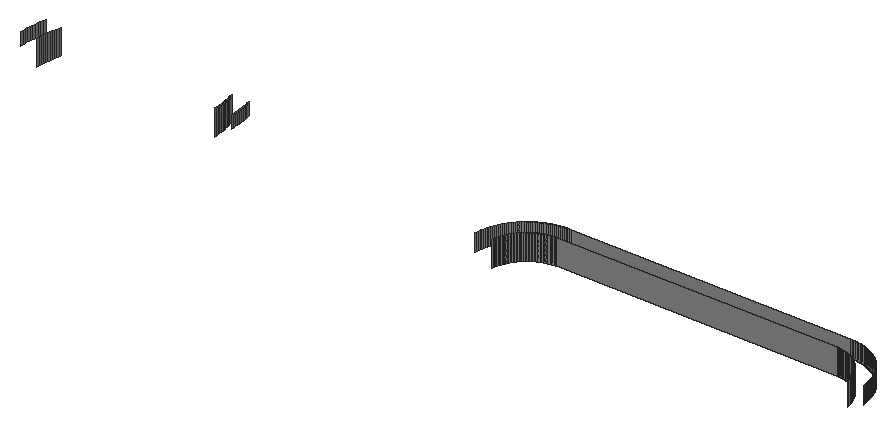
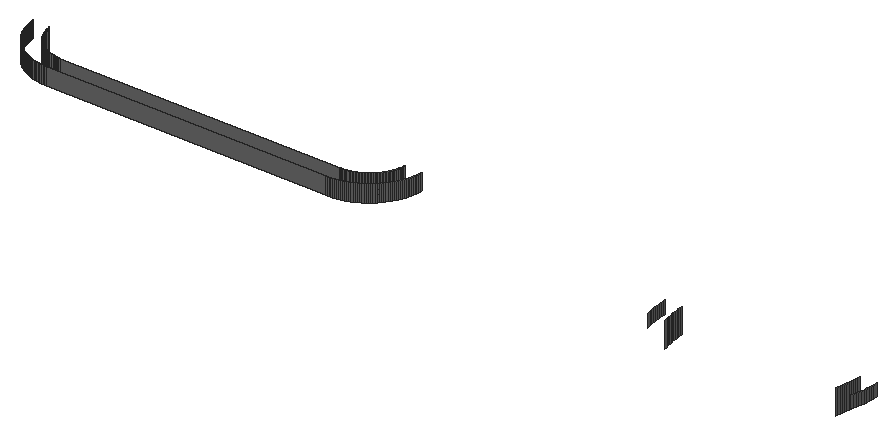
# SketchUp Ruby script. Lengths in inches.
U = 1.inch
M = Sketchup.active_model
def pt(a) = Geom::Point3d.new(a.map { |v| v * U })
def face(e, loops, mat)
  f = e.add_face(loops[0].map { |a| pt(a) })
  loops[1..].each { |l| e.add_face(l.map { |a| pt(a) }).erase! }
  f.material = f.back_material = mat if mat
  f
end
# faces: each face lists its corners as indices into pts; further lists are holes
def faces(e, pts, list, mat = nil) = list.each { |f| face(e, (f[0].is_a?(Array) ? f : [f]).map { |l| l.map { |i| pts[i] } }, mat) }
# xy, xz, yz: faces in a plane at the given z, y or x. An outline is a flat list of corners, or four numbers for a rectangle; further outlines are holes
def ring(l) = l.size == 4 ? [[l[0], l[1]], [l[2], l[1]], [l[2], l[3]], [l[0], l[3]]] : l.each_slice(2).to_a
def flat(e, list, mat, &to3) = list.each { |f| face(e, (f[0].is_a?(Array) ? f : [f]).map { |l| ring(l).map { |u, v| to3.(u, v) } }, mat) }
def xy(e, z, list, mat = nil) = flat(e, list, mat) { |x, y| [x, y, z] }
def xz(e, y, list, mat = nil) = flat(e, list, mat) { |x, z| [x, y, z] }
def yz(e, x, list, mat = nil) = flat(e, list, mat) { |y, z| [x, y, z] }
def lines(e, pts, list) = list.each { |a, b| e.add_line(pt(pts[a]), pt(pts[b])) }
# prism: a flat outline (further loops are holes) pulled along v
def prism(e, loops, v, mat = nil)
  f = face(e, loops, mat); d = Geom::Vector3d.new(v.map { |x| x * U })
  f.pushpull(f.normal.samedirection?(d) ? d.length : -d.length)
end
def box(e, o, s, mat = nil) = prism(e, [[o, [o[0] + s[0], o[1], o[2]], [o[0] + s[0], o[1] + s[1], o[2]], [o[0], o[1] + s[1], o[2]]]], [0, 0, s[2]], mat)
def at(x, y, z, deg = 0) = Geom::Transformation.translation(pt([x, y, z])) * Geom::Transformation.rotation(ORIGIN, Z_AXIS, deg.degrees)
def axes(o, x, y, z) = Geom::Transformation.new([*x, 0, *y, 0, *z, 0, *pt(o).to_a, 1])
def part(name) = M.definitions.add(name)
# library, detail: a bought-in or finely detailed component or shape, given as its bounding box
def library(name, o, s) = part(name).tap { |d| box(d.entities, o, s) }
def detail(e, o, s) = box(e.add_group.entities, o, s)
def put(e, d, t, mat = nil) = e.add_instance(d, t).tap { |i| i.material = mat if mat }
def group(e, t, mat = nil) = e.add_group.tap { |g| g.transformation = t; g.material = mat if mat }.entities
root = M.entities
M.materials.add("[Slate Light Tile]").color = [119, 119, 119]
M.materials.add("[Stone Coursed Rough]").color = [137, 137, 137]
xz(root,120,[[290.72,-2,291,4],[291,-2,357,4],[357,-2,357.28,4]],"[Stone Coursed Rough]")
xz(root,124,[[291,0,357,4]],"[Stone Coursed Rough]")
p = [[168.01,120.55,-3],[168.01,120.55,3],[168,120,3],[168,120,-3],[210,120,-3],[210,120,3],
  [209.99,120.55,3],[209.99,120.55,-3],[168.03,121.1,-3],[168.03,121.1,3],[209.97,121.1,3],[209.97,121.1,-3],
  [168.06,121.65,-3],[168.06,121.65,3],[209.94,121.65,3],[209.94,121.65,-3],[168.12,122.2,-3],[168.12,122.2,3],
  [209.88,122.2,3],[209.88,122.2,-3],[168.18,122.74,-3],[168.18,122.74,3],[209.82,122.74,3],[209.82,122.74,-3],
  [168.26,123.29,-3],[168.26,123.29,3],[209.74,123.29,3],[209.74,123.29,-3],[168.35,123.83,-3],[168.35,123.83,3],
  [209.65,123.83,3],[209.65,123.83,-3],[168.46,124.37,-3],[168.46,124.37,3],[209.54,124.37,3],[209.54,124.37,-3],
  [168.58,124.9,-3],[168.58,124.9,3],[209.42,124.9,3],[209.42,124.9,-3],[168.72,125.44,-3],[168.72,125.44,3],
  [209.28,125.44,3],[209.28,125.44,-3],[168.86,125.96,-3],[168.86,125.96,3],[209.14,125.96,3],[209.14,125.96,-3],
  [282.04,111.85,-2],[282.07,112.13,-2],[282.07,112.13,4],[282.04,111.85,4],[282.11,112.41,-2],[282.11,112.41,4],
  [365.89,112.41,-2],[365.93,112.13,-2],[365.93,112.13,4],[365.89,112.41,4],[282.16,112.6875,-2],[282.16,112.6875,4],
  [365.84,112.6875,-2],[365.84,112.6875,4],[282.22,112.96,-2],[282.22,112.96,4],[365.78,112.96,-2],[365.78,112.96,4],
  [282.28,113.24,-2],[282.28,113.24,4],[365.72,113.24,-2],[365.72,113.24,4],[282.36,113.51,-2],[282.36,113.51,4],
  [365.64,113.51,-2],[365.64,113.51,4],[282.44,113.78,-2],[282.44,113.78,4],[365.56,113.78,-2],[365.56,113.78,4],
  [282.53,114.05,-2],[282.53,114.05,4],[365.47,114.05,-2],[365.47,114.05,4],[282.63,114.3125,-2],[282.63,114.3125,4],
  [365.37,114.3125,-2],[365.37,114.3125,4],[282.74,114.57,-2],[282.74,114.57,4],[365.26,114.57,-2],[365.26,114.57,4],
  [282.86,114.83,-2],[282.86,114.83,4],[365.14,114.83,-2],[365.14,114.83,4],[282.98,115.09,-2],[282.98,115.09,4],
  [365.02,115.09,-2],[365.02,115.09,4],[283.11,115.34,-2],[283.11,115.34,4],[364.89,115.34,-2],[364.89,115.34,4],
  [283.25,115.58,-2],[283.25,115.58,4],[364.75,115.58,-2],[364.75,115.58,4],[283.4,115.82,-2],[283.4,115.82,4],
  [364.6,115.82,-2],[364.6,115.82,4],[283.56,116.06,-2],[283.56,116.06,4],[364.44,116.06,-2],[364.44,116.06,4],
  [283.72,116.29,-2],[283.72,116.29,4],[364.28,116.29,-2],[364.28,116.29,4],[283.89,116.52,-2],[283.89,116.52,4],
  [364.11,116.52,-2],[364.11,116.52,4],[284.07,116.74,-2],[284.07,116.74,4],[363.93,116.74,-2],[363.93,116.74,4],
  [284.25,116.95,-2],[284.25,116.95,4],[363.75,116.95,-2],[363.75,116.95,4],[284.4375,117.16,-2],[284.4375,117.16,4],
  [363.5625,117.16,-2],[363.5625,117.16,4],[284.64,117.36,-2],[284.64,117.36,4],[363.36,117.36,-2],[363.36,117.36,4],
  [284.84,117.5625,-2],[284.84,117.5625,4],[363.16,117.5625,-2],[363.16,117.5625,4],[285.05,117.75,-2],[285.05,117.75,4],
  [362.95,117.75,-2],[362.95,117.75,4],[285.26,117.93,-2],[285.26,117.93,4],[362.74,117.93,-2],[362.74,117.93,4],
  [285.48,118.11,-2],[285.48,118.11,4],[362.52,118.11,-2],[362.52,118.11,4],[285.71,118.28,-2],[285.71,118.28,4],
  [362.29,118.28,-2],[362.29,118.28,4],[285.94,118.44,-2],[285.94,118.44,4],[362.06,118.44,-2],[362.06,118.44,4],
  [286.18,118.6,-2],[286.18,118.6,4],[361.82,118.6,-2],[361.82,118.6,4],[286.42,118.75,-2],[286.42,118.75,4],
  [361.58,118.75,-2],[361.58,118.75,4],[286.66,118.89,-2],[286.66,118.89,4],[361.34,118.89,-2],[361.34,118.89,4],
  [286.91,119.02,-2],[286.91,119.02,4],[361.09,119.02,-2],[361.09,119.02,4],[287.17,119.14,-2],[287.17,119.14,4],
  [360.83,119.14,-2],[360.83,119.14,4],[287.43,119.26,-2],[287.43,119.26,4],[360.57,119.26,-2],[360.57,119.26,4],
  [287.6875,119.37,-2],[287.6875,119.37,4],[360.3125,119.37,-2],[360.3125,119.37,4],[287.95,119.47,-2],[287.95,119.47,4],
  [360.05,119.47,-2],[360.05,119.47,4],[288.22,119.56,-2],[288.22,119.56,4],[359.78,119.56,-2],[359.78,119.56,4],
  [288.49,119.64,-2],[288.49,119.64,4],[288.76,119.72,-2],[288.76,119.72,4],[359.24,119.72,-2],[359.51,119.64,-2],
  [359.51,119.64,4],[359.24,119.72,4],[289.04,119.78,-2],[289.04,119.78,4],[358.96,119.78,-2],[358.96,119.78,4],
  [289.3125,119.84,-2],[289.3125,119.84,4],[289.59,119.89,-2],[289.59,119.89,4],[358.41,119.89,-2],[358.6875,119.84,-2],
  [358.6875,119.84,4],[358.41,119.89,4],[289.87,119.93,-2],[289.87,119.93,4],[290.15,119.96,-2],[290.15,119.96,4],
  [357.85,119.96,-2],[358.13,119.93,-2],[358.13,119.93,4],[357.85,119.96,4],[290.43,119.98,-2],[290.43,119.98,4],
  [290.72,120,-2],[290.72,120,4],[357.28,120,-2],[357.57,119.98,-2],[357.57,119.98,4],[357.28,120,4],
  [278.06,112.22,0],[278.03,111.82,0],[278.03,111.82,4],[278.06,112.22,4],[369.97,111.82,0],[369.94,112.22,0],
  [369.94,112.22,4],[369.97,111.82,4],[278.1,112.63,0],[278.1,112.63,4],[369.9,112.63,0],[369.9,112.63,4],
  [278.16,113.03,0],[278.16,113.03,4],[369.84,113.03,0],[369.84,113.03,4],[278.23,113.4375,0],[278.23,113.4375,4],
  [369.77,113.4375,0],[369.77,113.4375,4],[278.3125,113.84,0],[278.3125,113.84,4],[369.6875,113.84,0],[369.6875,113.84,4],
  [278.41,114.23,0],[278.41,114.23,4],[369.59,114.23,0],[369.59,114.23,4],[278.52,114.625,0],[278.52,114.625,4],
  [369.48,114.625,0],[369.48,114.625,4],[278.64,115.02,0],[278.64,115.02,4],[369.36,115.02,0],[369.36,115.02,4],
  [278.77,115.4,0],[278.77,115.4,4],[369.23,115.4,0],[369.23,115.4,4],[278.91,115.79,0],[278.91,115.79,4],
  [369.09,115.79,0],[369.09,115.79,4],[279.07,116.16,0],[279.07,116.16,4],[368.93,116.16,0],[368.93,116.16,4],
  [279.24,116.54,0],[279.24,116.54,4],[368.76,116.54,0],[368.76,116.54,4],[279.42,116.9,0],[279.42,116.9,4],
  [368.58,116.9,0],[368.58,116.9,4],[279.61,117.26,0],[279.61,117.26,4],[368.39,117.26,0],[368.39,117.26,4],
  [279.81,117.62,0],[279.81,117.62,4],[368.19,117.62,0],[368.19,117.62,4],[280.02,117.97,0],[280.02,117.97,4],
  [367.98,117.97,0],[367.98,117.97,4],[280.25,118.31,0],[280.25,118.31,4],[367.75,118.31,0],[367.75,118.31,4],
  [280.48,118.64,0],[280.48,118.64,4],[367.52,118.64,0],[367.52,118.64,4],[280.73,118.97,0],[280.73,118.97,4],
  [367.27,118.97,0],[367.27,118.97,4],[280.98,119.29,0],[280.98,119.29,4],[367.02,119.29,0],[367.02,119.29,4],
  [281.25,119.6,0],[281.25,119.6,4],[366.75,119.6,0],[366.75,119.6,4],[281.52,119.9,0],[281.52,119.9,4],
  [366.48,119.9,0],[366.48,119.9,4],[281.81,120.19,0],[281.81,120.19,4],[366.19,120.19,0],[366.19,120.19,4],
  [164.01,120.65,0],[164,120,0],[164,120,3],[164.01,120.65,3],[214,120,0],[213.99,120.65,0],
  [213.99,120.65,3],[214,120,3],[282.1,120.48,0],[282.1,120.48,4],[365.9,120.48,0],[365.9,120.48,4],
  [282.4,120.75,0],[282.4,120.75,4],[365.6,120.75,0],[365.6,120.75,4],[164.03,121.31,0],[164.03,121.31,3],
  [213.97,121.31,0],[213.97,121.31,3],[282.71,121.02,0],[282.71,121.02,4],[365.29,121.02,0],[365.29,121.02,4],
  [283.03,121.27,0],[283.03,121.27,4],[364.97,121.27,0],[364.97,121.27,4],[164.08,121.96,0],[164.08,121.96,3],
  [213.92,121.96,0],[213.92,121.96,3],[283.36,121.52,0],[283.36,121.52,4],[364.64,121.52,0],[364.64,121.52,4],
  [283.69,121.75,0],[283.69,121.75,4],[364.31,121.75,0],[364.31,121.75,4],[284.03,121.98,0],[284.03,121.98,4],
  [363.97,121.98,0],[363.97,121.98,4],[164.14,122.61,0],[164.14,122.61,3],[213.86,122.61,0],[213.86,122.61,3],
  [284.38,122.19,0],[284.38,122.19,4],[363.62,122.19,0],[363.62,122.19,4],[284.74,122.39,0],[284.74,122.39,4],
  [363.26,122.39,0],[363.26,122.39,4],[285.1,122.58,0],[285.1,122.58,4],[362.9,122.58,0],[362.9,122.58,4],
  [164.21,123.26,0],[164.21,123.26,3],[213.79,123.26,0],[213.79,123.26,3],[285.46,122.76,0],[285.46,122.76,4],
  [362.54,122.76,0],[362.54,122.76,4],[285.84,122.93,0],[285.84,122.93,4],[362.16,122.93,0],[362.16,122.93,4],
  [286.21,123.09,0],[286.21,123.09,4],[361.79,123.09,0],[361.79,123.09,4],[286.6,123.23,0],[286.6,123.23,4],
  [361.4,123.23,0],[361.4,123.23,4],[286.98,123.36,0],[286.98,123.36,4],[361.02,123.36,0],[361.02,123.36,4],
  [164.31,123.91,0],[164.31,123.91,3],[213.69,123.91,0],[213.69,123.91,3],[287.375,123.48,0],[287.375,123.48,4],
  [360.625,123.48,0],[360.625,123.48,4],[287.77,123.59,0],[287.77,123.59,4],[360.23,123.59,0],[360.23,123.59,4],
  [288.16,123.6875,0],[288.16,123.6875,4],[359.84,123.6875,0],[359.84,123.6875,4],[288.5625,123.77,0],[288.5625,123.77,4],
  [359.4375,123.77,0],[359.4375,123.77,4],[288.97,123.84,0],[288.97,123.84,4],[289.37,123.9,0],[289.37,123.9,4],
  [359.03,123.84,0],[358.63,123.9,0],[358.63,123.9,4],[359.03,123.84,4],[164.42,124.56,0],[164.42,124.56,3],
  [213.58,124.56,0],[213.58,124.56,3],[289.78,123.94,0],[289.78,123.94,4],[290.18,123.97,0],[290.18,123.97,4],
  [358.22,123.94,0],[357.82,123.97,0],[357.82,123.97,4],[358.22,123.94,4],[290.59,123.99,0],[290.59,123.99,4],
  [291,124,0],[291,124,4],[357.41,123.99,0],[357,124,0],[357,124,4],[357.41,123.99,4],
  [164.55,125.2,0],[164.55,125.2,3],[213.45,125.2,0],[213.45,125.2,3],[164.69,125.84,0],[164.69,125.84,3],
  [213.31,125.84,0],[213.31,125.84,3],[164.85,126.47,0],[164.85,126.47,3]]
faces(root,p,[[0,1,2,3],[4,5,6,7],[8,9,1,0],[7,6,10,11],[12,13,9,8],[11,10,14,15],[16,17,13,12],[15,14,18,19],
  [20,21,17,16],[19,18,22,23],[24,25,21,20],[23,22,26,27],[28,29,25,24],[27,26,30,31],[32,33,29,28],[31,30,34,35],
  [36,37,33,32],[35,34,38,39],[40,41,37,36],[39,38,42,43],[44,45,41,40],[43,42,46,47],[330,331,332,333],[334,335,336,337],
  [346,330,333,347],[335,348,349,336],[358,346,347,359],[348,360,361,349],[374,358,359,375],[360,376,377,361],[390,374,375,391],[376,392,393,377],
  [414,390,391,415],[392,416,417,393],[442,414,415,443],[416,444,445,417],[462,442,443,463],[444,464,465,445],[466,462,463,467],[464,468,469,465],
  [470,466,467,471]],"[Slate Light Tile]")
faces(root,p,[[48,49,50,51],[49,52,53,50],[54,55,56,57],[52,58,59,53],[60,54,57,61],[58,62,63,59],[64,60,61,65],[62,66,67,63],
  [68,64,65,69],[66,70,71,67],[72,68,69,73],[70,74,75,71],[76,72,73,77],[74,78,79,75],[80,76,77,81],[78,82,83,79],
  [84,80,81,85],[82,86,87,83],[88,84,85,89],[86,90,91,87],[92,88,89,93],[90,94,95,91],[96,92,93,97],[94,98,99,95],
  [100,96,97,101],[98,102,103,99],[104,100,101,105],[102,106,107,103],[108,104,105,109],[106,110,111,107],[112,108,109,113],[110,114,115,111],
  [116,112,113,117],[114,118,119,115],[120,116,117,121],[118,122,123,119],[124,120,121,125],[122,126,127,123],[128,124,125,129],[126,130,131,127],
  [132,128,129,133],[130,134,135,131],[136,132,133,137],[134,138,139,135],[140,136,137,141],[138,142,143,139],[144,140,141,145],[142,146,147,143],
  [148,144,145,149],[146,150,151,147],[152,148,149,153],[150,154,155,151],[156,152,153,157],[154,158,159,155],[160,156,157,161],[158,162,163,159],
  [164,160,161,165],[162,166,167,163],[168,164,165,169],[166,170,171,167],[172,168,169,173],[170,174,175,171],[176,172,173,177],[174,178,179,175],
  [180,176,177,181],[178,182,183,179],[184,180,181,185],[182,186,187,183],[188,184,185,189],[186,190,191,187],[192,188,189,193],[190,194,195,191],
  [196,192,193,197],[194,198,199,195],[198,200,201,199],[202,203,204,205],[203,196,197,204],[200,206,207,201],[208,202,205,209],[206,210,211,207],
  [210,212,213,211],[214,215,216,217],[215,208,209,216],[212,218,219,213],[218,220,221,219],[222,223,224,225],[223,214,217,224],[220,226,227,221],
  [226,228,229,227],[230,231,232,233],[231,222,225,232],[234,235,236,237],[238,239,240,241],[242,234,237,243],[239,244,245,240],[246,242,243,247],
  [244,248,249,245],[250,246,247,251],[248,252,253,249],[254,250,251,255],[252,256,257,253],[258,254,255,259],[256,260,261,257],[262,258,259,263],
  [260,264,265,261],[266,262,263,267],[264,268,269,265],[270,266,267,271],[268,272,273,269],[274,270,271,275],[272,276,277,273],[278,274,275,279],
  [276,280,281,277],[282,278,279,283],[280,284,285,281],[286,282,283,287],[284,288,289,285],[290,286,287,291],[288,292,293,289],[294,290,291,295],
  [292,296,297,293],[298,294,295,299],[296,300,301,297],[302,298,299,303],[300,304,305,301],[306,302,303,307],[304,308,309,305],[310,306,307,311],
  [308,312,313,309],[314,310,311,315],[312,316,317,313],[318,314,315,319],[316,320,321,317],[322,318,319,323],[320,324,325,321],[326,322,323,327],
  [324,328,329,325],[338,326,327,339],[328,340,341,329],[342,338,339,343],[340,344,345,341],[350,342,343,351],[344,352,353,345],[354,350,351,355],
  [352,356,357,353],[362,354,355,363],[356,364,365,357],[366,362,363,367],[364,368,369,365],[370,366,367,371],[368,372,373,369],[378,370,371,379],
  [372,380,381,373],[382,378,379,383],[380,384,385,381],[386,382,383,387],[384,388,389,385],[394,386,387,395],[388,396,397,389],[398,394,395,399],
  [396,400,401,397],[402,398,399,403],[400,404,405,401],[406,402,403,407],[404,408,409,405],[410,406,407,411],[408,412,413,409],[418,410,411,419],
  [412,420,421,413],[422,418,419,423],[420,424,425,421],[426,422,423,427],[424,428,429,425],[430,426,427,431],[428,432,433,429],[434,430,431,435],
  [436,434,435,437],[438,439,440,441],[432,438,441,433],[446,436,437,447],[448,446,447,449],[450,451,452,453],[439,450,453,440],[454,448,449,455],
  [456,454,455,457],[458,459,460,461],[451,458,461,452]],"[Stone Coursed Rough]")
